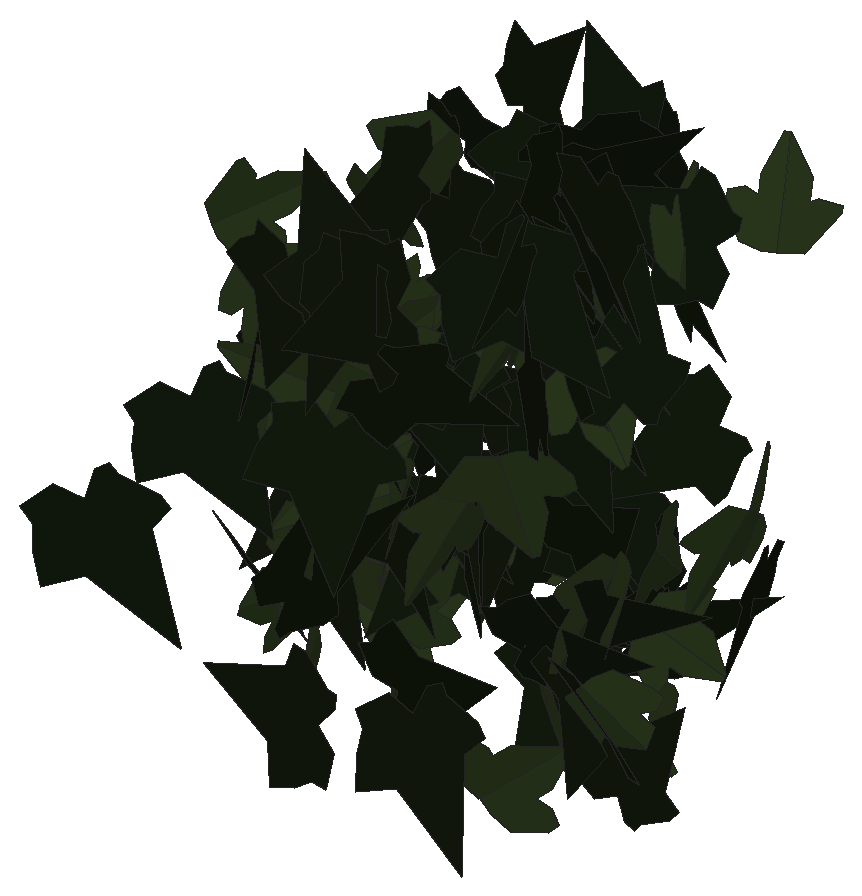
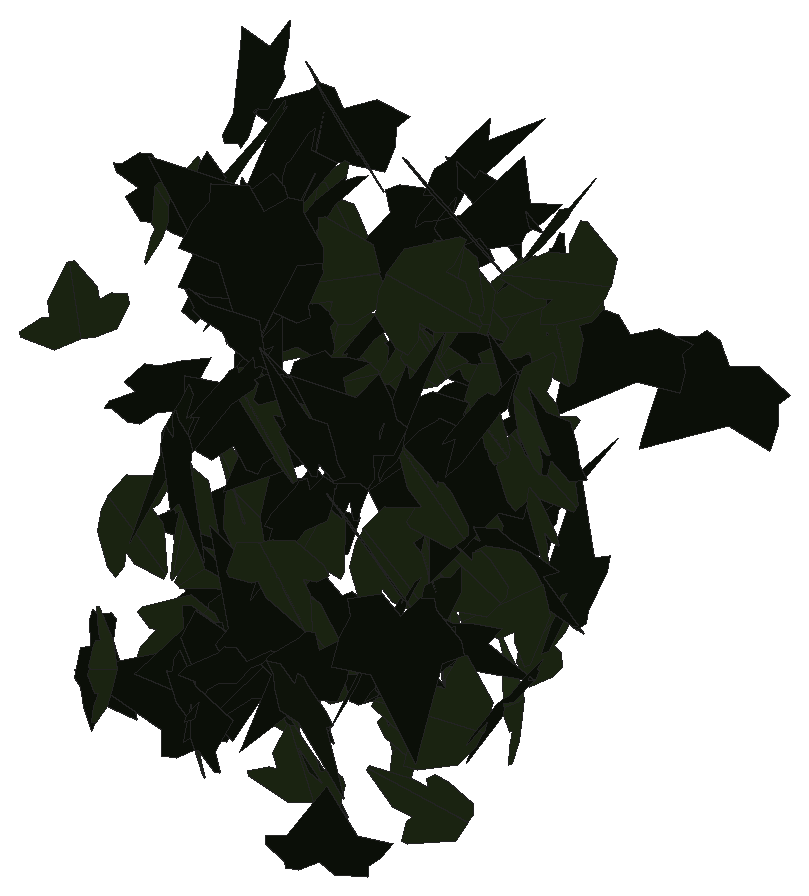
# SketchUp Ruby script. Lengths in inches.
U = 1.inch
M = Sketchup.active_model
def pt(a) = Geom::Point3d.new(a.map { |v| v * U })
def face(e, loops, mat)
  f = e.add_face(loops[0].map { |a| pt(a) })
  loops[1..].each { |l| e.add_face(l.map { |a| pt(a) }).erase! }
  f.material = f.back_material = mat if mat
  f
end
# faces: each face lists its corners as indices into pts; further lists are holes
def faces(e, pts, list, mat = nil) = list.each { |f| face(e, (f[0].is_a?(Array) ? f : [f]).map { |l| l.map { |i| pts[i] } }, mat) }
# xy, xz, yz: faces in a plane at the given z, y or x. An outline is a flat list of corners, or four numbers for a rectangle; further outlines are holes
def ring(l) = l.size == 4 ? [[l[0], l[1]], [l[2], l[1]], [l[2], l[3]], [l[0], l[3]]] : l.each_slice(2).to_a
def flat(e, list, mat, &to3) = list.each { |f| face(e, (f[0].is_a?(Array) ? f : [f]).map { |l| ring(l).map { |u, v| to3.(u, v) } }, mat) }
def xy(e, z, list, mat = nil) = flat(e, list, mat) { |x, y| [x, y, z] }
def xz(e, y, list, mat = nil) = flat(e, list, mat) { |x, z| [x, y, z] }
def yz(e, x, list, mat = nil) = flat(e, list, mat) { |y, z| [x, y, z] }
def lines(e, pts, list) = list.each { |a, b| e.add_line(pt(pts[a]), pt(pts[b])) }
# prism: a flat outline (further loops are holes) pulled along v
def prism(e, loops, v, mat = nil)
  f = face(e, loops, mat); d = Geom::Vector3d.new(v.map { |x| x * U })
  f.pushpull(f.normal.samedirection?(d) ? d.length : -d.length)
end
def box(e, o, s, mat = nil) = prism(e, [[o, [o[0] + s[0], o[1], o[2]], [o[0] + s[0], o[1] + s[1], o[2]], [o[0], o[1] + s[1], o[2]]]], [0, 0, s[2]], mat)
def at(x, y, z, deg = 0) = Geom::Transformation.translation(pt([x, y, z])) * Geom::Transformation.rotation(ORIGIN, Z_AXIS, deg.degrees)
def axes(o, x, y, z) = Geom::Transformation.new([*x, 0, *y, 0, *z, 0, *pt(o).to_a, 1])
def part(name) = M.definitions.add(name)
# library, detail: a bought-in or finely detailed component or shape, given as its bounding box
def library(name, o, s) = part(name).tap { |d| box(d.entities, o, s) }
def detail(e, o, s) = box(e.add_group.entities, o, s)
def put(e, d, t, mat = nil) = e.add_instance(d, t).tap { |i| i.material = mat if mat }
def group(e, t, mat = nil) = e.add_group.tap { |g| g.transformation = t; g.material = mat if mat }.entities
root = M.entities
M.materials.add("efeu1").color = [18, 25, 13]
M.materials.add("efeu2").color = [43, 57, 29]
c1 = part("ivyleaf_9")
p = [[1.54,2.16,1.25],[1.36,2.04,1.19],[-0.21,0.99,0.68],[-0.71,1.11,0.82],[-0.85,0.86,0.67],[-0.8,0.17,0.21],
  [-0.9,-0.01,0.1],[-0.67,-0.16,-0.02],[-0.08,-0.08,-0.05],[-0.03,-0.6,-0.4],[0.65,-0.88,-0.66],[0.83,-0.6,-0.49],
  [1.29,-0.42,-0.43],[1.8125,-0.07,-0.26],[1.21,0.44,0.15]]
faces(c1.entities,p,[[0,1,2,3,4,5,6,7,8,9,10,11,12,13,14]],"efeu1")
c2 = part("ivyleaf_10")
p = [[0,0.5,-0.03],[-0.0625,2.02,-0.43],[-0.19,2.01,-0.46],[-0.54,1.05,-0.29],[-0.52,0.625,-0.18],[-0.83,0.76,-0.28],
  [-1.16,0.64,-0.33],[-1.15,0.33,-0.24],[-0.77,-0.39,0.02],[-0.3,-0.51,0.16],[0.04,-0.48,0.23],[-0.02,2.01,-0.4375],
  [-0.06,2.01,-0.43],[0.04,-0.49,0.23],[0.67,-0.49,0.14],[1.38,0.36,-0.2],[1.375,0.51,-0.24],[0.81,0.65,-0.19],
  [0.62,0.59,-0.15],[0.6,1.09,-0.28],[0.5,1.23,-0.31]]
faces(c2.entities,p,[[0,1,2,3,4,5,6,7,8,9,10],[11,12,0,13,14,15,16,17,18,19,20]],"efeu2")
put(root,c1,axes([544.79,132.79,174.2],[0.32665,-0.691,-0.20454],[-0.08602,0.18558,-0.76432],[0.71548,0.33779,0.00149]))
put(root,c2,axes([544.875,130.26,182.26],[-0.10482,-0.27405,0.82991],[0.24404,0.79343,0.29283],[-0.83922,0.26496,-0.0185]))
put(root,c2,axes([545.08,131.8,180.1],[0.34201,-0.6783,0.58779],[0.23307,-0.54032,-0.75913],[0.86675,0.41294,-0.0278]))
put(root,c1,axes([545.53,135.1875,176.66],[0.5205,0.48408,-0.60741],[-0.46695,-0.38927,-0.71037],[-0.62067,0.69881,0.02506]))
put(root,c1,axes([544.99,131.3,178.86],[-0.41775,0.36828,0.74908],[0.52759,-0.53262,0.55609],[0.64684,0.67228,0.03021]))
put(root,c2,axes([544.85,132.29,176.3],[-0.60293,0.22787,-0.73093],[0.68901,-0.2442,-0.64448],[-0.33385,-0.91551,-0.01002]))
put(root,c2,axes([545.71,131.43,173.19],[0.391,-0.30598,0.88595],[-0.63763,0.61676,0.49442],[-0.68699,-0.74659,0.04535]))
put(root,c1,axes([545.63,137.55,172.43],[-0.72496,-0.23257,0.3128],[0.31086,0.05351,0.76027],[-0.23515,0.78775,0.0407]))
put(root,c1,axes([545.82,133.9,175.59],[-0.71357,-0.37116,0.27644],[-0.23744,-0.14246,-0.80417],[0.39724,-0.75187,0.01591]))
put(root,c2,axes([545.21,133.8,173.89],[-0.09445,-0.48182,0.82601],[0.21894,0.79709,0.48998],[-0.93087,0.23636,0.03143]))
put(root,c1,axes([545.02,125.77,178.29],[-0.25004,-0.33732,-0.96585],[0.64294,0.72159,-0.41846],[0.79579,-0.68898,0.03461]))
put(root,c1,axes([545.4375,135.66,180.91],[-0.03598,-0.16594,0.94635],[-0.21703,-0.92113,-0.16976],[0.93595,-0.21998,-0.00299]))
put(root,c1,axes([545.95,132.05,176.85],[-0.97168,-0.14808,-0.00848],[0.00843,0.001,-0.9829],[0.14808,-0.97172,0.00028]))
put(root,c2,axes([545.46,131.13,174.32],[-0.15842,0.25694,0.88052],[0.30073,-0.82962,0.29619],[0.86654,0.33489,0.05818]))
put(root,c2,axes([545.76,131.04,178.5625],[-0.13049,-0.67748,0.49323],[-0.10722,-0.48157,-0.68983],[0.83111,-0.16849,-0.01155]))
put(root,c2,axes([545.59,130.39,181.3125],[0.38205,0.86265,-0.25554],[-0.0994,-0.23546,-0.94345],[-0.89419,0.39474,-0.00431]))
put(root,c2,axes([545.1,134.32,172.2],[0.42605,-0.04888,-0.73488],[0.72708,0.16328,0.41067],[0.11743,-0.83361,0.12353]))
put(root,c1,axes([545.3,130.44,174.84],[0.86471,-0.49175,-0.28372],[0.2671,-0.10379,0.99395],[-0.50097,-0.90413,0.04021]))
put(root,c2,axes([545.26,134.08,178.53],[0.5865,-0.21706,-0.6099],[0.58021,-0.18878,0.62514],[-0.28714,-0.82482,0.01743]))
put(root,c2,axes([545.91,138.74,179.52],[0.81152,0.15388,-0.26291],[-0.25927,-0.04384,-0.82597],[-0.15992,0.85192,0.00499]))
put(root,c1,axes([545.49,137.87,181.51],[-0.27272,0.3486,0.68757],[0.44852,-0.52142,0.44227],[0.62698,0.52464,-0.01731]))
put(root,c1,axes([545.21,136.55,181.18],[0.19202,-0.19658,0.77799],[0.64255,-0.44151,-0.27015],[0.48066,0.66874,0.05033]))
put(root,c1,axes([546.47,137.25,175.77],[-0.46268,0.66311,0.16397],[-0.09474,0.13383,-0.80857],[-0.67648,-0.47228,0.00109]))
put(root,c1,axes([545.77,132.03,180.16],[0.29657,-0.72446,-0.39418],[-0.14642,0.36598,-0.78281],[0.81165,0.33073,0.00281]))
put(root,c1,axes([545.64,133.74,176],[0.79158,-0.47803,-0.10684],[-0.08931,0.05879,-0.92471],[0.48161,0.79659,0.00413]))
put(root,c2,axes([545.63,132.52,176.19],[0.48902,-0.02601,-0.62997],[0.62934,-0.02843,0.4897],[-0.03841,-0.79699,0.00309]))
put(root,c1,axes([545.73,127.93,179.72],[-0.1566,-0.55605,-0.80167],[0.40776,0.70032,-0.5654],[0.88634,-0.42042,0.11847]))
put(root,c1,axes([546.4,134.86,177.59],[-0.65043,0.63245,0.13165],[0.08372,-0.10272,0.9071],[0.64056,0.65562,0.01512]))
put(root,c1,axes([546.16,129.66,181.44],[-0.22563,-0.00366,-0.85863],[0.75175,-0.4298,-0.19572],[-0.41488,-0.7768,0.11233]))
put(root,c1,axes([546.55,131.42,178.38],[0.34791,0.87464,0.18615],[0.06216,0.17561,-0.94127],[-0.89206,0.35335,0.00702]))
put(root,c2,axes([547.1,130.83,178.92],[0.02922,0.07757,-1.0189],[-0.68702,0.75604,0.03785],[0.75643,0.68368,0.07374]))
put(root,c2,axes([546.73,133.49,182.92],[-0.17507,-0.56918,0.78491],[-0.12274,-0.77818,-0.59168],[0.96176,-0.20292,0.06737]))
put(root,c2,axes([546.16,133.34,173.18],[-0.74071,-0.27616,0.56116],[0.52496,0.19828,0.79051],[-0.33996,0.90787,-0.00196]))
put(root,c1,axes([546.875,134.2,174.62],[-0.64327,-0.5386,0.2061],[-0.16053,-0.12932,-0.83897],[0.55389,-0.66299,-0.00379]))
put(root,c2,axes([546.82,131.91,182.61],[-0.85848,0.2685,0.05403],[-0.05221,0.01407,-0.89949],[-0.26885,-0.86007,0.00216]))
put(root,c2,axes([546.79,132.625,176.23],[0.59185,-0.73086,0.1577],[0.1008,-0.12129,-0.94045],[0.74086,0.60037,0.00198]))
put(root,c2,axes([547.5,129.125,180.19],[-0.26312,-0.05485,-0.84838],[-0.82929,-0.17897,0.26877],[-0.18717,0.87002,0.0018]))
put(root,c2,axes([546.74,136.56,173.15],[0.79185,0.19229,-0.11739],[0.10167,0.07781,0.81326],[0.20104,-0.79671,0.05109]))
put(root,c2,axes([546.78,129.67,176.65],[0.74139,-0.46828,0.11897],[0.10154,-0.06201,-0.87689],[0.47236,0.74831,0.00178]))
put(root,c1,axes([546.77,133.77,175.85],[0.54527,-0.43197,-0.62968],[-0.42631,0.46972,-0.6914],[0.63352,0.68788,0.0767]))
put(root,c1,axes([546.54,132.49,175.58],[0.43922,-0.67093,-0.0204],[-0.01121,0.01705,-0.80191],[0.67115,0.43937,-0.00004]))
put(root,c1,axes([547.46,135.61,173.3125],[-0.645,0.3125,-0.45456],[-0.41849,0.17843,0.71647],[0.35937,0.76864,0.01848]))
put(root,c2,axes([547.27,130.92,176.91],[-0.09701,0.03472,0.93901],[-0.12552,-0.93602,0.02164],[0.93123,-0.12254,0.10074]))
put(root,c1,axes([546.93,136.08,175.84],[0.1132,-0.31602,-0.74694],[-0.17195,0.72768,-0.33393],[0.7926,0.203,0.03423]))
put(root,c1,axes([546.78,129.46,181.94],[-0.04606,-0.80776,0.5954],[0.10288,-0.59669,-0.80155],[0.99819,0.02422,0.11009]))
put(root,c1,axes([546.95,134.33,175.24],[-0.27649,-0.04987,-0.81742],[0.81852,-0.04446,-0.27415],[-0.02623,-0.86177,0.06145]))
put(root,c1,axes([547.21,135.96,179.24],[0.25928,-0.45785,-0.63289],[-0.30937,0.55213,-0.52617],[0.71727,0.40365,0.00183]))
put(root,c1,axes([547.49,136.06,181.85],[-0.49111,-0.66212,0.06401],[-0.03105,-0.05666,-0.82433],[0.66448,-0.49201,0.00879]))
put(root,c1,axes([547.19,128.89,175.78],[0.10299,0.1337,1.01729],[0.69465,0.74337,-0.16803],[-0.75513,0.70206,-0.01582]))
put(root,c1,axes([547.86,129.76,182.07],[-0.61412,-0.59294,0.28239],[0.21262,0.1863,0.85355],[-0.62138,0.64976,0.01297]))
put(root,c1,axes([547.4,133.36,182.05],[0.45121,-0.53112,-0.52878],[-0.25095,0.47452,-0.69075],[0.7062,0.50797,0.09239]))
put(root,c1,axes([547.54,134.24,178.4],[0.03724,0.31494,0.82233],[-0.19084,-0.80062,0.31527],[0.85965,-0.19137,0.03437]))
put(root,c1,axes([548.21,131.22,183.82],[-0.78456,0.3526,0.08163],[-0.07592,0.03021,-0.86014],[-0.35387,-0.78821,0.00355]))
put(root,c1,axes([548.36,138.65,181.13],[0.08424,0.0511,-0.878],[-0.87902,0.03366,-0.08237],[0.02868,0.88139,0.05405]))
put(root,c1,axes([547.73,134.23,175.99],[-0.64196,-0.22742,-0.54099],[0.5181,0.15695,-0.68077],[0.27563,-0.82471,0.01962]))
put(root,c2,axes([547.42,131.92,180.37],[0.50372,-0.34877,-0.56935],[0.53134,-0.2225,0.60638],[-0.40432,-0.7269,0.08757]))
put(root,c2,axes([547.94,132.16,171.88],[-0.00105,0.01749,-0.83667],[-0.12594,-0.82714,-0.01713],[-0.82732,0.12589,0.00367]))
put(root,c2,axes([547.95,134.58,180.7],[-0.17553,-0.17666,0.8406],[0.19736,-0.84331,-0.13602],[0.83598,0.16199,0.20861]))
put(root,c2,axes([548.14,132.6,176.27],[-0.0621,-0.8137,0.51781],[-0.02028,-0.51767,-0.81591],[0.96428,-0.06329,0.01619]))
put(root,c2,axes([547.89,130.28,180.32],[-0.01203,-0.38747,0.96378],[0.02718,0.9634,0.38766],[-1.0384,0.02971,-0.00102]))
put(root,c1,axes([547.74,132.26,179.41],[-0.32437,-0.60678,-0.67825],[0.32837,0.5935,-0.688],[0.84875,-0.46152,0.00697]))
put(root,c1,axes([548.3,131,180.05],[-0.64141,-0.55624,0.03278],[-0.02405,-0.02229,-0.84901],[0.55669,-0.64186,0.00108]))
put(root,c1,axes([548.1,129.03,179.4],[-0.39013,-0.83718,-0.37572],[0.14643,0.34623,-0.92354],[0.90587,-0.41652,-0.01252]))
put(root,c1,axes([548.91,136.42,182.47],[-0.83389,0.0537,-0.27122],[-0.27129,0.0075,0.83557],[0.05339,0.87686,0.00946]))
put(root,c2,axes([548.56,130.21,173.89],[0.43212,-0.80605,-0.48884],[-0.17541,0.45961,-0.91291],[0.92624,0.46309,0.05517]))
put(root,c2,axes([548.03,130.13,180.23],[-0.50442,-0.44969,-0.84006],[0.63756,0.5471,-0.67569],[0.70812,-0.81291,0.00996]))
put(root,c1,axes([548.6,127.8,174.12],[0.05362,-0.93985,-0.20129],[0.06725,-0.19744,0.93979],[-0.95881,-0.06641,0.05466]))
put(root,c1,axes([548.48,129.125,182.73],[-0.78038,-0.20119,-0.38935],[0.38326,0.07237,-0.80557],[0.21257,-0.86911,0.02305]))
put(root,c2,axes([548.79,133.5625,177.02],[-0.06373,-0.52352,-0.73971],[0.15716,0.72391,-0.52588],[0.89249,-0.16486,0.03978]))
put(root,c1,axes([548.5625,136.48,181.59],[0.38881,-0.57137,-0.53863],[-0.24091,0.48526,-0.68865],[0.74736,0.45367,0.05823]))
put(root,c1,axes([548.6875,136.08,175.02],[-0.03659,-0.55673,-0.61185],[0.14821,0.59813,-0.55311],[0.81385,-0.13396,0.07321]))
put(root,c1,axes([548.87,136.07,174.49],[-0.08927,-0.80801,-0.15941],[0.01898,0.15828,-0.81292],[0.82336,-0.09125,0.00146]))
put(root,c1,axes([549.26,129.27,182.33],[-0.30446,-0.40887,0.87701],[-0.38909,-0.79006,-0.50341],[0.88596,-0.48748,0.0803]))
put(root,c1,axes([549.7,136.48,173.66],[-0.05177,0.06678,0.83715],[-0.4357,0.71489,-0.08397],[-0.71794,-0.43866,-0.00941]))
put(root,c1,axes([549.6,134.38,183.85],[0.43052,0.78696,-0.27204],[-0.13844,-0.23433,-0.89698],[-0.82106,0.45215,0.0086]))
put(root,c2,axes([549.89,134.46,179.9],[0.64216,-0.32282,-0.60773],[-0.5362,0.28627,-0.71864],[0.43131,0.83651,0.01141]))
put(root,c1,axes([548.99,134.86,174.72],[-0.18792,-0.10209,0.90296],[0.71284,-0.58843,0.08182],[0.56358,0.71022,0.19759]))
put(root,c1,axes([549.23,133.29,179.13],[-0.08692,-0.34994,-0.84075],[0.35247,0.76582,-0.35519],[0.83969,-0.35768,0.06207]))
put(root,c1,axes([549.35,134.45,182.01],[0.81784,0.26641,0.14666],[-0.13924,-0.04607,0.86014],[0.27036,-0.82961,-0.00066]))
put(root,c1,axes([549.77,136.65,180.19],[0.6511,-0.29975,-0.51463],[-0.46044,0.23028,-0.71666],[0.37775,0.79734,0.01351]))
put(root,c1,axes([549.5625,128.75,181.19],[0.0135,0.1341,-0.89414],[0.27584,0.85099,0.1318],[0.86103,-0.27473,-0.0282]))
put(root,c1,axes([550.2,133.75,173.36],[-0.82406,-0.48288,-0.08674],[0.07353,0.04608,-0.95511],[0.48506,-0.82733,-0.00257]))
put(root,c1,axes([550.11,134.59,178.84],[0.69556,-0.20347,0.51118],[-0.49182,0.1394,0.7247],[-0.24662,-0.85186,-0.00351]))
put(root,c2,axes([549.47,131.63,181.41],[0.20868,0.06065,0.89339],[0.66408,0.60489,-0.19619],[-0.60069,0.68979,0.09348]))
put(root,c2,axes([550.65,132.48,172.31],[-0.54322,0.5754,-0.56238],[-0.39635,0.39914,0.79123],[0.70019,0.67234,0.01158]))
put(root,c1,axes([549.98,133.21,183.78],[0.11086,-0.24209,-0.83674],[0.58702,-0.60241,0.25207],[-0.64354,-0.59121,0.08579]))
put(root,c1,axes([549.95,132.71,182.99],[0.01876,-0.95995,0.10687],[0.01212,-0.10665,-0.96008],[0.96581,0.01998,0.00997]))
put(root,c1,axes([549.59,129.12,174.59],[0.13747,-0.08827,0.88895],[0.73639,-0.49797,-0.16332],[0.50572,0.7491,-0.00382]))
put(root,c1,axes([549.77,134.22,183.02],[0.62389,0.67196,-0.27281],[0.18636,0.19924,0.91694],[0.70088,-0.65113,-0.00097]))
put(root,c2,axes([550.94,137.53,174.73],[0.2864,-0.37503,0.75007],[-0.48832,0.56978,0.47134],[-0.68176,-0.56566,-0.02251]))
put(root,c1,axes([550.74,134.4,173.68],[-0.22682,0.62464,-0.5285],[-0.24314,0.47221,0.66245],[0.78127,0.32831,0.05273]))
put(root,c1,axes([550.46,132.9375,182.29],[-0.008,-0.53688,0.69339],[0.07227,-0.69147,-0.53456],[0.87396,0.05227,0.05055]))
put(root,c2,axes([550.75,131.29,181.92],[0.16006,-0.49896,0.81623],[0.22354,-0.78516,-0.5238],[0.93017,0.27455,-0.01457]))
put(root,c2,axes([550.43,130.82,172.02],[-0.6267,-0.30094,0.6971],[0.63605,0.28557,0.6951],[-0.41468,0.89283,0.01264]))
put(root,c1,axes([550.3125,134.97,173.2],[0.32597,0.03667,0.9143],[0.8504,0.34617,-0.31707],[-0.33781,0.90685,0.08406]))
put(root,c2,axes([550.29,131.41,181.62],[0.04114,-0.10916,0.8964],[0.89979,0.08079,-0.03146],[-0.07631,0.8937,0.11234]))
put(root,c2,axes([551.05,130.34,179.07],[-0.83552,-0.50603,-0.18202],[0.15464,0.09602,-0.97681],[0.51506,-0.84971,-0.00199]))
put(root,c1,axes([551.58,130.01,184],[-0.77474,0.23162,-0.36199],[0.34978,-0.0937,-0.80857],[-0.24968,-0.84999,-0.00951]))
put(root,c1,axes([550.61,131.48,174.73],[0.36741,-0.1867,0.87126],[0.82701,-0.27934,-0.40861],[0.33167,0.90335,0.05372]))
put(root,c2,axes([551.6,132.41,176.01],[0.15092,-0.77413,0.62807],[0.10667,-0.61904,-0.78863],[0.99115,0.18449,-0.01076]))
put(root,c2,axes([551.57,134.35,172.49],[0.56637,-0.63545,0.04914],[0.03276,-0.03662,-0.85122],[0.6365,0.56732,0.00009]))
put(root,c2,axes([551.4375,134.31,174.19],[0.14755,0.56416,0.62273],[0.13689,0.60767,-0.58295],[-0.82905,0.20074,0.01458]))
put(root,c1,axes([551.3,131.57,180.21],[-0.35352,-0.31316,-0.77527],[0.60207,0.48874,-0.47196],[0.5802,-0.69797,0.01737]))
put(root,c1,axes([551.23,132.81,183.875],[0.40459,-0.91344,0.16816],[0.06086,-0.15696,-0.999],[0.92679,0.40906,-0.00781]))
put(root,c1,axes([551.25,129.94,183.65],[0.00887,-0.57967,-0.91706],[0.27262,0.88886,-0.5592],[1.05009,-0.22587,0.15292]))
put(root,c1,axes([551.21,131.65,175.44],[0.21338,0.50362,-0.77703],[0.2917,0.72023,0.54692],[0.87882,-0.36134,0.00713]))
put(root,c1,axes([551.86,136.8,174.55],[-0.3664,0.30158,-0.71827],[0.56314,-0.44591,-0.47449],[-0.53826,-0.6718,-0.00749]))
put(root,c1,axes([551.6,126.99,175.6],[0.15422,-0.90626,-0.43034],[-0.085,0.42203,-0.91922],[0.99964,0.1757,-0.01177]))
put(root,c1,axes([551.62,132.24,174.03],[-0.052,-0.82143,0.53342],[0.06576,-0.5359,-0.81883],[0.97722,-0.00764,0.08349]))
put(root,c1,axes([551.97,132.88,180.53],[0.5962,-0.65239,0.21976],[-0.14523,0.16498,0.88377],[-0.67291,-0.61363,0.00397]))
put(root,c2,axes([552.12,133.39,176.47],[0.05931,-0.60517,-0.65708],[-0.06984,0.65337,-0.60806],[0.89057,0.09154,-0.00392]))
put(root,c1,axes([552.09,132.3125,173.08],[0.5723,-0.78694,0.12747],[-0.07311,0.10444,0.97303],[-0.79383,-0.57695,0.00228]))
put(root,c1,axes([551.85,131.41,181.38],[0.64451,-0.55899,-0.33011],[-0.24842,0.21739,-0.85315],[0.59978,0.69072,0.00136]))
put(root,c2,axes([552.11,136.875,181.67],[0.5141,0.66701,-0.19705],[0.0993,0.17214,0.84174],[0.68838,-0.52297,0.02573]))
put(root,c1,axes([552.47,129.48,180.91],[0.01474,-0.50522,0.9314],[-0.00102,0.93148,0.50528],[-1.0596,-0.00792,0.01247]))
put(root,c2,axes([552.3,132.04,176.27],[0.59487,-0.76866,-0.10225],[-0.0581,0.08433,-0.97195],[0.77326,0.59767,0.00564]))
put(root,c1,axes([553.03,133.76,183],[-0.57299,-0.28515,-0.64426],[-0.55069,-0.3367,0.6388],[-0.43945,0.79374,0.03953]))
put(root,c2,axes([552.54,133.48,182.66],[0.02875,0.6044,-0.66477],[-0.10019,0.66312,0.59856],[0.89285,0.05495,0.08858]))
put(root,c1,axes([552.71,134.26,178.86],[-0.61227,-0.46556,0.47357],[-0.35129,-0.31958,-0.76835],[0.56357,-0.70499,0.03556]))
put(root,c2,axes([552.66,134.89,176.45],[0.02217,-0.77693,0.45023],[0.00342,-0.45029,-0.7772],[0.89795,0.02089,-0.00815]))
put(root,c2,axes([552.34,131.07,181.1],[0.55898,0.55203,0.36239],[0.25835,0.25413,-0.78562],[-0.60772,0.61579,-0.00065]))
put(root,c2,axes([552.46,131.35,174.375],[-0.64777,-0.04385,-0.63204],[0.63197,0.01927,-0.64904],[0.04485,-0.90483,0.01681]))
put(root,c1,axes([553.1,131.1875,181.01],[-0.88657,0.1692,0.27892],[0.26779,-0.08382,0.90205],[0.18631,0.92562,0.0307]))
put(root,c1,axes([552.41,131.05,183.89],[0.12176,-0.52444,0.80331],[0.30166,-0.74775,-0.5339],[0.91069,0.31781,0.06944]))
put(root,c1,axes([552.79,131.46,172.57],[-0.37954,0.13403,0.72992],[0.62443,-0.38538,0.39544],[0.40105,0.72686,0.07507]))
